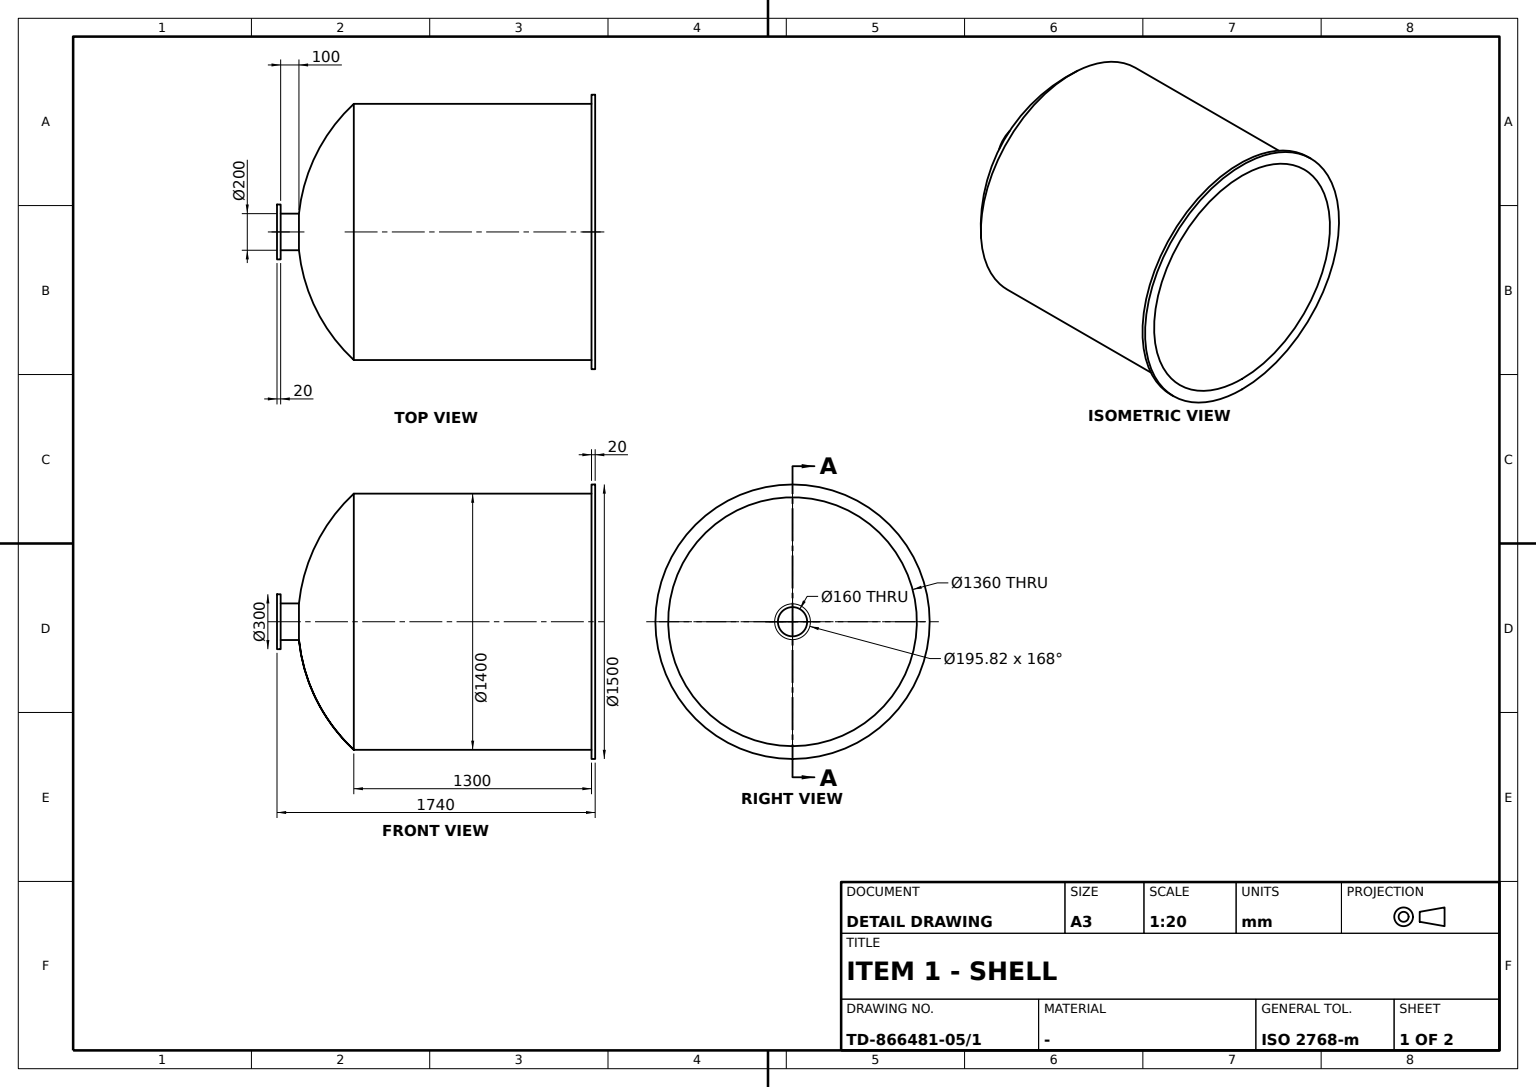
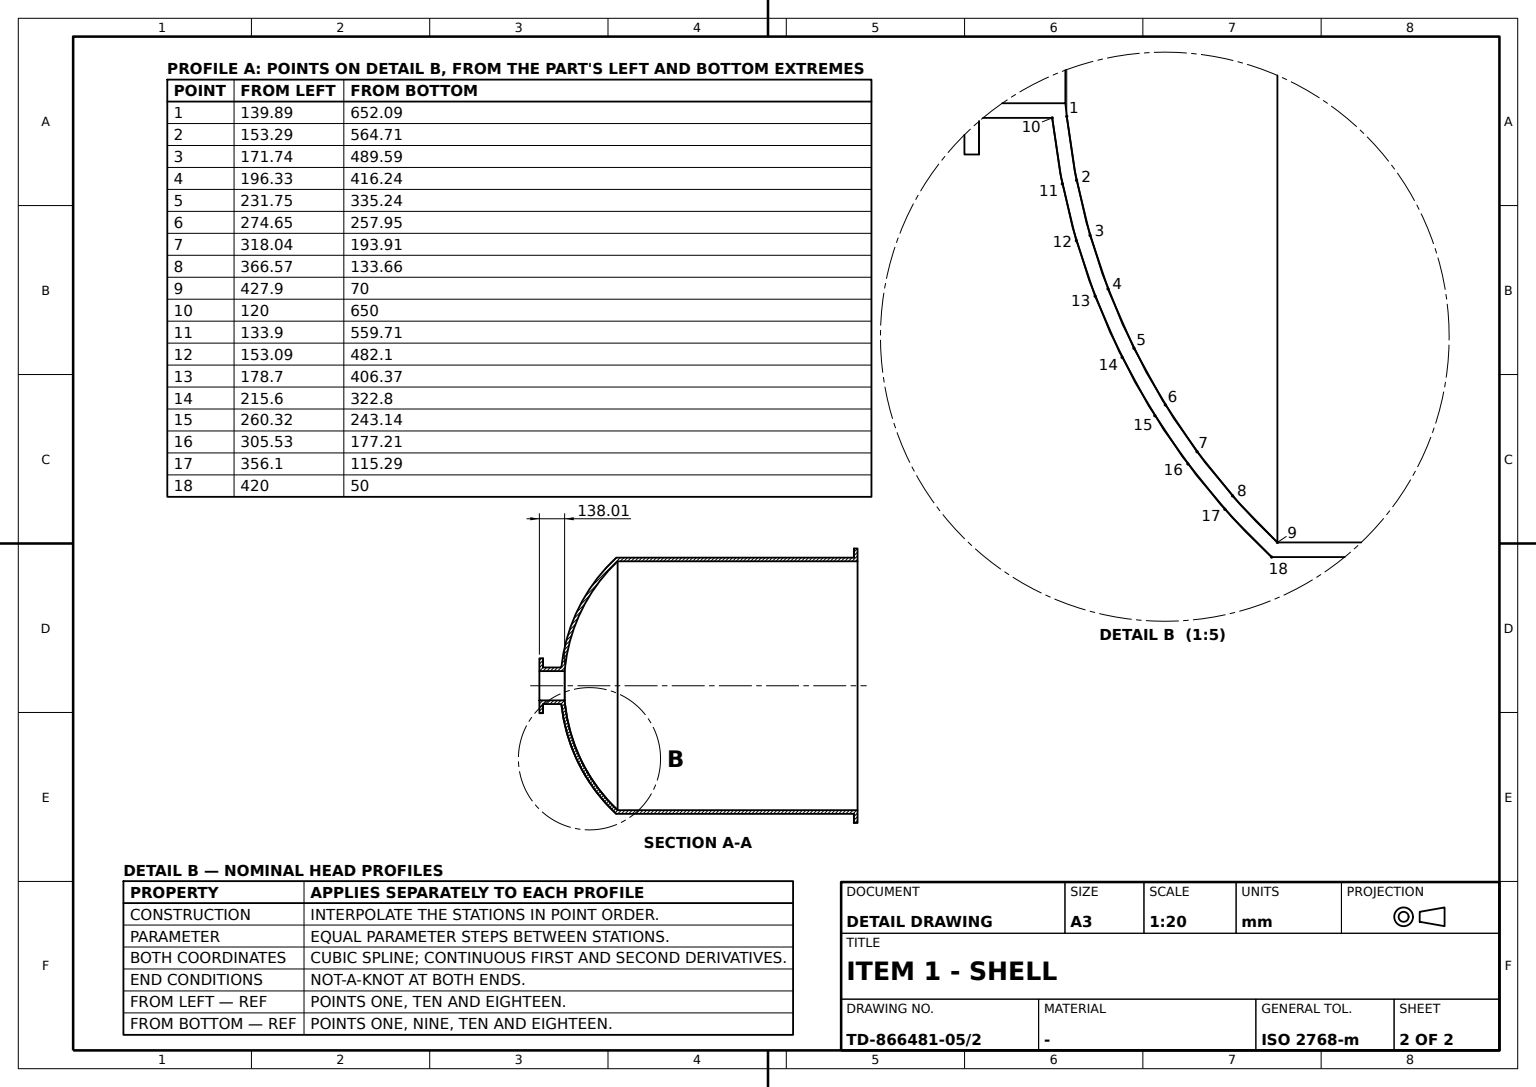
ISO-10303-21;
HEADER;
FILE_DESCRIPTION((''),'2;1');
FILE_NAME('','',(''),(''),'','','');
FILE_SCHEMA(('AUTOMOTIVE_DESIGN'));
ENDSEC;
DATA;
#1=APPLICATION_CONTEXT('');
#2=PRODUCT_CONTEXT('',#1,'mechanical');
#3=PRODUCT('','','',(#2));
#4=PRODUCT_DEFINITION_FORMATION('','',#3);
#5=PRODUCT_DEFINITION_CONTEXT('',#1,'design');
#6=PRODUCT_DEFINITION('','',#4,#5);
#7=PRODUCT_DEFINITION_SHAPE('','',#6);
#8=(LENGTH_UNIT()NAMED_UNIT(*)SI_UNIT(.MILLI.,.METRE.));
#9=(NAMED_UNIT(*)PLANE_ANGLE_UNIT()SI_UNIT($,.RADIAN.));
#10=(NAMED_UNIT(*)SI_UNIT($,.STERADIAN.)SOLID_ANGLE_UNIT());
#11=UNCERTAINTY_MEASURE_WITH_UNIT(LENGTH_MEASURE(0.005),#8,'distance_accuracy_value','');
#12=(GEOMETRIC_REPRESENTATION_CONTEXT(3)GLOBAL_UNCERTAINTY_ASSIGNED_CONTEXT((#11))GLOBAL_UNIT_ASSIGNED_CONTEXT((#8,#9,#10))REPRESENTATION_CONTEXT('',''));
#13=CARTESIAN_POINT('',(100.,0.,120.));
#14=VERTEX_POINT('',#13);
#15=CARTESIAN_POINT('',(0.,0.,120.));
#16=DIRECTION('',(0.,0.,1.));
#17=DIRECTION('',(1.,0.,0.));
#18=AXIS2_PLACEMENT_3D('',#15,#16,#17);
#19=CIRCLE('',#18,100.);
#20=EDGE_CURVE('',#14,#14,#19,.T.);
#21=ORIENTED_EDGE('',*,*,#20,.F.);
#22=EDGE_LOOP('',(#21));
#23=FACE_BOUND('',#22,.T.);
#24=CARTESIAN_POINT('',(100.,0.,20.));
#25=VERTEX_POINT('',#24);
#26=CARTESIAN_POINT('',(0.,0.,20.));
#27=AXIS2_PLACEMENT_3D('',#26,#16,#17);
#28=CIRCLE('',#27,100.);
#29=EDGE_CURVE('',#25,#25,#28,.T.);
#30=ORIENTED_EDGE('',*,*,#29,.T.);
#31=EDGE_LOOP('',(#30));
#32=FACE_BOUND('',#31,.T.);
#33=CARTESIAN_POINT('',(0.,0.,860.));
#34=AXIS2_PLACEMENT_3D('',#33,#16,#17);
#35=CYLINDRICAL_SURFACE('',#34,100.);
#36=ADVANCED_FACE('',(#23,#32),#35,.T.);
#37=CARTESIAN_POINT('',(80.,0.,138.005235));
#38=VERTEX_POINT('',#37);
#39=CARTESIAN_POINT('',(0.,0.,138.005235));
#40=AXIS2_PLACEMENT_3D('',#39,#16,#17);
#41=CIRCLE('',#40,80.);
#42=EDGE_CURVE('',#38,#38,#41,.T.);
#43=ORIENTED_EDGE('',*,*,#42,.F.);
#44=EDGE_LOOP('',(#43));
#45=FACE_BOUND('',#44,.T.);
#46=CARTESIAN_POINT('',(97.906304,0.,139.890109));
#47=VERTEX_POINT('',#46);
#48=CARTESIAN_POINT('',(0.,0.,139.890109));
#49=AXIS2_PLACEMENT_3D('',#48,#16,#17);
#50=CIRCLE('',#49,97.906304);
#51=EDGE_CURVE('',#47,#47,#50,.T.);
#52=ORIENTED_EDGE('',*,*,#51,.T.);
#53=EDGE_LOOP('',(#52));
#54=FACE_BOUND('',#53,.T.);
#55=CONICAL_SURFACE('',#40,80.,1.465919388);
#56=ADVANCED_FACE('',(#45,#54),#55,.F.);
#57=ORIENTED_EDGE('',*,*,#20,.T.);
#58=EDGE_LOOP('',(#57));
#59=FACE_BOUND('',#58,.T.);
#60=CARTESIAN_POINT('',(700.,0.,420.));
#61=VERTEX_POINT('',#60);
#62=CARTESIAN_POINT('',(0.,0.,420.));
#63=AXIS2_PLACEMENT_3D('',#62,#16,#17);
#64=CIRCLE('',#63,700.);
#65=EDGE_CURVE('',#61,#61,#64,.T.);
#66=ORIENTED_EDGE('',*,*,#65,.F.);
#67=EDGE_LOOP('',(#66));
#68=FACE_BOUND('',#67,.T.);
#69=CARTESIAN_POINT('',(0.,0.,1070.));
#70=AXIS2_PLACEMENT_3D('',#69,#16,#17);
#71=SPHERICAL_SURFACE('',#70,955.248659);
#72=ADVANCED_FACE('',(#59,#68),#71,.T.);
#73=ORIENTED_EDGE('',*,*,#42,.T.);
#74=EDGE_LOOP('',(#73));
#75=FACE_BOUND('',#74,.T.);
#76=CARTESIAN_POINT('',(80.,0.,0.));
#77=VERTEX_POINT('',#76);
#78=CARTESIAN_POINT('',(0.,0.,0.));
#79=AXIS2_PLACEMENT_3D('',#78,#16,#17);
#80=CIRCLE('',#79,80.);
#81=EDGE_CURVE('',#77,#77,#80,.T.);
#82=ORIENTED_EDGE('',*,*,#81,.F.);
#83=EDGE_LOOP('',(#82));
#84=FACE_BOUND('',#83,.T.);
#85=CYLINDRICAL_SURFACE('',#34,80.);
#86=ADVANCED_FACE('',(#75,#84),#85,.F.);
#87=CARTESIAN_POINT('',(680.,0.,1740.));
#88=VERTEX_POINT('',#87);
#89=CARTESIAN_POINT('',(0.,0.,1740.));
#90=AXIS2_PLACEMENT_3D('',#89,#16,#17);
#91=CIRCLE('',#90,680.);
#92=EDGE_CURVE('',#88,#88,#91,.T.);
#93=ORIENTED_EDGE('',*,*,#92,.F.);
#94=EDGE_LOOP('',(#93));
#95=FACE_BOUND('',#94,.T.);
#96=CARTESIAN_POINT('',(750.,0.,1740.));
#97=VERTEX_POINT('',#96);
#98=CIRCLE('',#90,750.);
#99=EDGE_CURVE('',#97,#97,#98,.T.);
#100=ORIENTED_EDGE('',*,*,#99,.T.);
#101=EDGE_LOOP('',(#100));
#102=FACE_BOUND('',#101,.T.);
#103=CARTESIAN_POINT('',(0.,-680.,1740.));
#104=AXIS2_PLACEMENT_3D('',#103,#16,#17);
#105=PLANE('',#104);
#106=ADVANCED_FACE('',(#95,#102),#105,.T.);
#107=ORIENTED_EDGE('',*,*,#65,.T.);
#108=EDGE_LOOP('',(#107));
#109=FACE_BOUND('',#108,.T.);
#110=CARTESIAN_POINT('',(700.,0.,1720.));
#111=VERTEX_POINT('',#110);
#112=CARTESIAN_POINT('',(0.,0.,1720.));
#113=AXIS2_PLACEMENT_3D('',#112,#16,#17);
#114=CIRCLE('',#113,700.);
#115=EDGE_CURVE('',#111,#111,#114,.T.);
#116=ORIENTED_EDGE('',*,*,#115,.F.);
#117=EDGE_LOOP('',(#116));
#118=FACE_BOUND('',#117,.T.);
#119=CYLINDRICAL_SURFACE('',#34,700.);
#120=ADVANCED_FACE('',(#109,#118),#119,.T.);
#121=ORIENTED_EDGE('',*,*,#92,.T.);
#122=EDGE_LOOP('',(#121));
#123=FACE_BOUND('',#122,.T.);
#124=CARTESIAN_POINT('',(680.,0.,427.901835));
#125=VERTEX_POINT('',#124);
#126=CARTESIAN_POINT('',(0.,0.,427.901835));
#127=AXIS2_PLACEMENT_3D('',#126,#16,#17);
#128=CIRCLE('',#127,680.);
#129=EDGE_CURVE('',#125,#125,#128,.T.);
#130=ORIENTED_EDGE('',*,*,#129,.F.);
#131=EDGE_LOOP('',(#130));
#132=FACE_BOUND('',#131,.T.);
#133=CYLINDRICAL_SURFACE('',#34,680.);
#134=ADVANCED_FACE('',(#123,#132),#133,.F.);
#135=CARTESIAN_POINT('',(150.,0.,0.));
#136=VERTEX_POINT('',#135);
#137=CIRCLE('',#79,150.);
#138=EDGE_CURVE('',#136,#136,#137,.T.);
#139=ORIENTED_EDGE('',*,*,#138,.F.);
#140=EDGE_LOOP('',(#139));
#141=FACE_BOUND('',#140,.T.);
#142=ORIENTED_EDGE('',*,*,#81,.T.);
#143=EDGE_LOOP('',(#142));
#144=FACE_BOUND('',#143,.T.);
#145=CARTESIAN_POINT('',(0.,-100.,0.));
#146=AXIS2_PLACEMENT_3D('',#145,#16,#17);
#147=PLANE('',#146);
#148=ADVANCED_FACE('',(#141,#144),#147,.F.);
#149=ORIENTED_EDGE('',*,*,#29,.F.);
#150=EDGE_LOOP('',(#149));
#151=FACE_BOUND('',#150,.T.);
#152=CARTESIAN_POINT('',(150.,0.,20.));
#153=VERTEX_POINT('',#152);
#154=CIRCLE('',#27,150.);
#155=EDGE_CURVE('',#153,#153,#154,.T.);
#156=ORIENTED_EDGE('',*,*,#155,.T.);
#157=EDGE_LOOP('',(#156));
#158=FACE_BOUND('',#157,.T.);
#159=CARTESIAN_POINT('',(0.,-150.,20.));
#160=AXIS2_PLACEMENT_3D('',#159,#16,#17);
#161=PLANE('',#160);
#162=ADVANCED_FACE('',(#151,#158),#161,.T.);
#163=ORIENTED_EDGE('',*,*,#155,.F.);
#164=EDGE_LOOP('',(#163));
#165=FACE_BOUND('',#164,.T.);
#166=ORIENTED_EDGE('',*,*,#138,.T.);
#167=EDGE_LOOP('',(#166));
#168=FACE_BOUND('',#167,.T.);
#169=CYLINDRICAL_SURFACE('',#34,150.);
#170=ADVANCED_FACE('',(#165,#168),#169,.T.);
#171=ORIENTED_EDGE('',*,*,#115,.T.);
#172=EDGE_LOOP('',(#171));
#173=FACE_BOUND('',#172,.T.);
#174=CARTESIAN_POINT('',(750.,0.,1720.));
#175=VERTEX_POINT('',#174);
#176=CIRCLE('',#113,750.);
#177=EDGE_CURVE('',#175,#175,#176,.T.);
#178=ORIENTED_EDGE('',*,*,#177,.F.);
#179=EDGE_LOOP('',(#178));
#180=FACE_BOUND('',#179,.T.);
#181=CARTESIAN_POINT('',(0.,-700.,1720.));
#182=AXIS2_PLACEMENT_3D('',#181,#16,#17);
#183=PLANE('',#182);
#184=ADVANCED_FACE('',(#173,#180),#183,.F.);
#185=ORIENTED_EDGE('',*,*,#129,.T.);
#186=EDGE_LOOP('',(#185));
#187=FACE_BOUND('',#186,.T.);
#188=ORIENTED_EDGE('',*,*,#51,.F.);
#189=EDGE_LOOP('',(#188));
#190=FACE_BOUND('',#189,.T.);
#191=SPHERICAL_SURFACE('',#70,935.248659);
#192=ADVANCED_FACE('',(#187,#190),#191,.F.);
#193=ORIENTED_EDGE('',*,*,#99,.F.);
#194=EDGE_LOOP('',(#193));
#195=FACE_BOUND('',#194,.T.);
#196=ORIENTED_EDGE('',*,*,#177,.T.);
#197=EDGE_LOOP('',(#196));
#198=FACE_BOUND('',#197,.T.);
#199=CYLINDRICAL_SURFACE('',#34,750.);
#200=ADVANCED_FACE('',(#195,#198),#199,.T.);
#201=CLOSED_SHELL('',(#36,#56,#72,#86,#106,#120,#134,#148,#162,#170,#184,#192,#200));
#202=MANIFOLD_SOLID_BREP('',#201);
#203=ADVANCED_BREP_SHAPE_REPRESENTATION('',(#202),#12);
#204=SHAPE_DEFINITION_REPRESENTATION(#7,#203);
ENDSEC;
END-ISO-10303-21;
